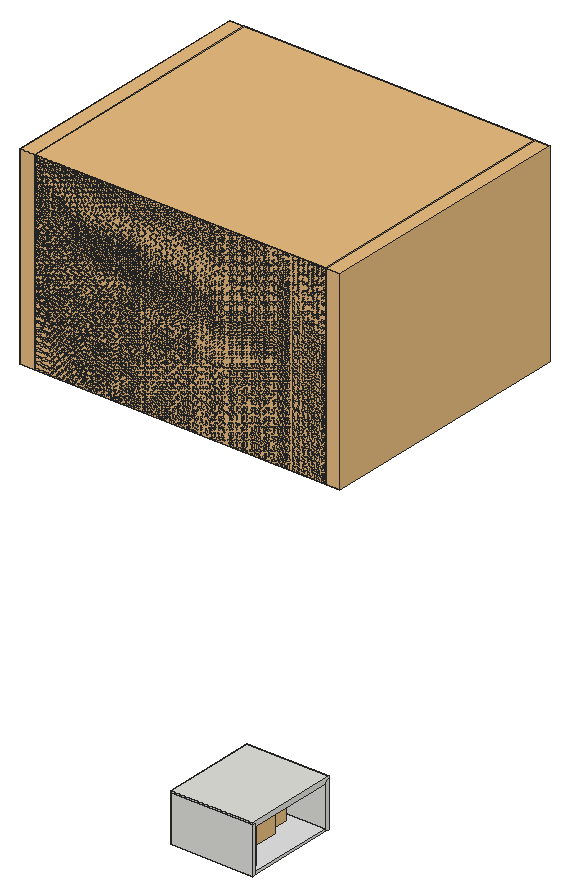
# SketchUp Ruby script. Lengths in inches.
U = 1.inch
M = Sketchup.active_model
def pt(a) = Geom::Point3d.new(a.map { |v| v * U })
def face(e, loops, mat)
  f = e.add_face(loops[0].map { |a| pt(a) })
  loops[1..].each { |l| e.add_face(l.map { |a| pt(a) }).erase! }
  f.material = f.back_material = mat if mat
  f
end
# faces: each face lists its corners as indices into pts; further lists are holes
def faces(e, pts, list, mat = nil) = list.each { |f| face(e, (f[0].is_a?(Array) ? f : [f]).map { |l| l.map { |i| pts[i] } }, mat) }
# xy, xz, yz: faces in a plane at the given z, y or x. An outline is a flat list of corners, or four numbers for a rectangle; further outlines are holes
def ring(l) = l.size == 4 ? [[l[0], l[1]], [l[2], l[1]], [l[2], l[3]], [l[0], l[3]]] : l.each_slice(2).to_a
def flat(e, list, mat, &to3) = list.each { |f| face(e, (f[0].is_a?(Array) ? f : [f]).map { |l| ring(l).map { |u, v| to3.(u, v) } }, mat) }
def xy(e, z, list, mat = nil) = flat(e, list, mat) { |x, y| [x, y, z] }
def xz(e, y, list, mat = nil) = flat(e, list, mat) { |x, z| [x, y, z] }
def yz(e, x, list, mat = nil) = flat(e, list, mat) { |y, z| [x, y, z] }
def lines(e, pts, list) = list.each { |a, b| e.add_line(pt(pts[a]), pt(pts[b])) }
# prism: a flat outline (further loops are holes) pulled along v
def prism(e, loops, v, mat = nil)
  f = face(e, loops, mat); d = Geom::Vector3d.new(v.map { |x| x * U })
  f.pushpull(f.normal.samedirection?(d) ? d.length : -d.length)
end
def box(e, o, s, mat = nil) = prism(e, [[o, [o[0] + s[0], o[1], o[2]], [o[0] + s[0], o[1] + s[1], o[2]], [o[0], o[1] + s[1], o[2]]]], [0, 0, s[2]], mat)
def at(x, y, z, deg = 0) = Geom::Transformation.translation(pt([x, y, z])) * Geom::Transformation.rotation(ORIGIN, Z_AXIS, deg.degrees)
def axes(o, x, y, z) = Geom::Transformation.new([*x, 0, *y, 0, *z, 0, *pt(o).to_a, 1])
def part(name) = M.definitions.add(name)
# library, detail: a bought-in or finely detailed component or shape, given as its bounding box
def library(name, o, s) = part(name).tap { |d| box(d.entities, o, s) }
def detail(e, o, s) = box(e.add_group.entities, o, s)
def put(e, d, t, mat = nil) = e.add_instance(d, t).tap { |i| i.material = mat if mat }
def group(e, t, mat = nil) = e.add_group.tap { |g| g.transformation = t; g.material = mat if mat }.entities
root = M.entities
M.materials.add("1466 AP 9476 Soft Whisper").color = [230, 233, 224]
M.materials.add("1472 AP 9469 Black Sea").color = [67, 75, 78]
M.materials.add("[Carrera Marble]").color = [207, 207, 207]
M.materials.add("[Granite Light Gray]").color = [49, 48, 47]
M.materials.add("[Marble Carrara Gold Floor Tile]").color = [229, 229, 229]
M.materials.add("[Stone Vein Gray]").color = [94, 94, 94]
M.materials.add("[Translucent Glass Blue]").color = [163, 215, 254]
M.materials.add("[Wood Veneer 01]").color = [83, 56, 38]
M.materials.add("[Wood Veneer 01]1").color = [74, 43, 22]
M.materials.add("[Wood Veneer 01]2").color = [120, 70, 37]
c1 = library("Object02",[-606.68,-655.71,-190.21],[1149.33,653.61,1636.06])
c2 = part("skp42")
put(c2.entities,c1,at(0,0,0))
c3 = part("Senza")
put(c3.entities,c2,at(-166.13,607.08,194.25))
c4 = library("kitchen+utensil",[-39.88,-27.4,0],[79.77,28.4,32.96])
c5 = library("1\#1",[-14.37,-13.42,0],[27.79,27.79,26.46])
c6 = library("ACCESS \#17",[0,0,0],[12.33,19.09,15.22])
c7 = library("AS-120-mm",[0,0,0],[63,4.72,48])
c8 = library("Potted Plant",[-13.58,-10.04,0],[38.83,39.25,67.18])
c9 = library("Mi & Gei Hardware - Brass Towel Ring",[0,0,0],[7.7,2.76,18.21])
c10 = library("DC3A\#1",[-17.72,-4.29,0],[35.44,8.58,13.65])
c11 = library("ILVE HP75C",[-22.61,-16.47,-1.74],[45.22,32.94,3.48])
c12 = library("11",[-1.9375,-1.9375,-28],[4,4,28])
c13 = library("Kitchen Tray Decor",[57.57,5.21,10.61],[18.31,18.31,13.72])
c14 = part("1")
box(c14.entities,[-20,0,0],[20,51,0.39])
c15 = library("2",[-1,-0.25,-0.25],[1,51.5,32.375])
c16 = part("5")
box(c16.entities,[0,-0.25,-0.25],[0.5,45,11.6875])
c17 = part("6")
box(c17.entities,[0,-0.25,-0.25],[0.5,45,15.9375])
c18 = library("תנור פולגור",[76.05,-2.36,7.75],[23.79,26.38,23.66])
c19 = library("\#1",[-189.34,-482.08,-290.58],[543.74,599.14,350.96])
c20 = part("Mixer\#1")
put(c20.entities,c19,at(-26.63,749.7,289.625))
c21 = library("ACCESS \#28",[0,0,-0.01],[22.01,8.97,21.09])
c22 = library("Kitchen+Sink",[0,0,-9.45],[39.37,19.69,22.29])
c23 = library("Drawer fronts",[0,0,0],[1.57,26.54,41.66])
c24 = library("French door refrigerator",[0,0,0],[35.5,29.25,69.5])
c25 = library("Group\#61",[-3.28,0,-3.2],[6.56,11.56,7.1])
c26 = library("Group1\#6",[-3.97,-4.36,4.58],[7.94,7.57,1.92])
c27 = library("Group2\#4",[-28.125,-19.52,30.85],[56.26,48.19,42.76])
c28 = part("215693")
put(c28.entities,c25,axes([0,0,0],[6.23163,0,0],[0,0,6.44624],[0,-6.23163,0]))
put(c28.entities,c26,axes([0,0.01,17.77],[2.3609,0,0],[0,2.52448,0],[0,0,1.96338]))
put(c28.entities,c27,axes([0.01,0.44,706.86],[14.88915,0,0],[0,14.88915,0],[0,0,12.38215]))
c29 = library("angular chimney",[0,0,0],[18.55,32.4,33.35])
c30 = library("oats",[14.82,-39.71,51.49],[19.78,4.73,8.06])
c31 = library("Group\#4",[0,0,0],[177,126,2])
c32 = library("Group\#6",[0,0,0],[0.5,124,34])
c33 = library("Group\#13",[0,0,0],[23.39,15.89,14.65])
c34 = library("Group\#43",[0,0,0],[27,126,29])
c35 = library("Group\#45",[0,0,-0.25],[18.5,126,21.25])
c36 = library("Group\#46",[0,0,-58.43],[152.74,148.09,107])
c37 = library("Group\#51",[0,0,0],[21.5,54,111])
c38 = library("Group\#53",[0,-18,0],[48,18,50])
c39 = library("Group\#59",[-5,-18,0],[6,18,71])
c40 = library("Group\#79",[0,-1,0],[23.9375,1,23.9375])
c41 = library("Group\#78",[0,0,-2.62],[198,180,7.62])
c42 = part("Group282\#1")
box(c42.entities,[-102,-4.5,0],[1,9,0.5])
c43 = part("Group283\#1")
box(c43.entities,[-100.5,-4.5,0],[1,9,0.5])
c44 = part("Group284\#1")
box(c44.entities,[-99,-4.5,0],[1,9,0.5])
c45 = part("Group285\#1")
box(c45.entities,[-97.5,-4.5,0],[1,9,0.5])
c46 = part("Group286\#1")
box(c46.entities,[-96,-4.5,0],[1,9,0.5])
c47 = part("Group287\#1")
box(c47.entities,[-94.5,-4.5,0],[1,9,0.5])
c48 = part("Group288\#1")
box(c48.entities,[-93,-4.5,0],[1,9,0.5])
c49 = part("Group289\#1")
box(c49.entities,[-91.5,-4.5,0],[1,9,0.5])
c50 = part("Group290\#1")
box(c50.entities,[-90,-4.5,0],[1,9,0.5])
c51 = part("Group291\#1")
box(c51.entities,[-88.5,-4.5,0],[1,9,0.5])
c52 = part("Group292\#1")
box(c52.entities,[-87,-4.5,0],[1,9,0.5])
c53 = part("Group293\#1")
box(c53.entities,[-85.5,-4.5,0],[1,9,0.5])
c54 = part("Group294\#1")
box(c54.entities,[-84,-4.5,0],[1,9,0.5])
c55 = part("Group295\#1")
box(c55.entities,[-82.5,-4.5,0],[1,9,0.5])
c56 = part("Group296\#1")
box(c56.entities,[-81,-4.5,0],[1,9,0.5])
c57 = part("Group297\#1")
box(c57.entities,[-79.5,-4.5,0],[1,9,0.5])
c58 = part("Group298\#1")
box(c58.entities,[-78,-4.5,0],[1,9,0.5])
c59 = part("Group299\#1")
box(c59.entities,[-76.5,-4.5,0],[1,9,0.5])
c60 = part("Group300\#1")
box(c60.entities,[-75,-4.5,0],[1,9,0.5])
c61 = part("Group301\#1")
box(c61.entities,[-73.5,-4.5,0],[1,9,0.5])
c62 = part("Group302\#1")
box(c62.entities,[-72,-4.5,0],[1,9,0.5])
c63 = part("Group303\#1")
box(c63.entities,[-70.5,-4.5,0],[1,9,0.5])
c64 = part("Group304\#1")
box(c64.entities,[-69,-4.5,0],[1,9,0.5])
c65 = part("Group305\#1")
box(c65.entities,[-67.5,-4.5,0],[1,9,0.5])
c66 = part("Group306\#1")
box(c66.entities,[-66,-4.5,0],[1,9,0.5])
c67 = part("Group307\#1")
box(c67.entities,[-64.5,-4.5,0],[1,9,0.5])
c68 = part("Group308\#1")
box(c68.entities,[-63,-4.5,0],[1,9,0.5])
c69 = part("Group309\#1")
box(c69.entities,[-61.5,-4.5,0],[1,9,0.5])
c70 = part("Group310\#1")
box(c70.entities,[-60,-4.5,0],[1,9,0.5])
c71 = part("Group311\#1")
box(c71.entities,[-58.5,-4.5,0],[1,9,0.5])
c72 = part("Group312\#1")
box(c72.entities,[-57,-4.5,0],[1,9,0.5])
c73 = part("Group313\#1")
box(c73.entities,[-55.5,-4.5,0],[1,9,0.5])
c74 = part("Group314\#1")
box(c74.entities,[-54,-4.5,0],[1,9,0.5])
c75 = part("Group315\#1")
box(c75.entities,[-52.5,-4.5,0],[1,9,0.5])
c76 = part("Group316\#1")
box(c76.entities,[-51,-4.5,0],[1,9,0.5])
c77 = part("Group317\#1")
box(c77.entities,[-49.5,-4.5,0],[1,9,0.5])
c78 = part("Group318\#1")
box(c78.entities,[-48,-4.5,0],[1,9,0.5])
c79 = part("Group319\#1")
box(c79.entities,[-46.5,-4.5,0],[1,9,0.5])
c80 = part("Group320\#1")
box(c80.entities,[-45,-4.5,0],[1,9,0.5])
c81 = part("Group321\#1")
box(c81.entities,[-43.5,-4.5,0],[1,9,0.5])
c82 = part("Group322\#1")
box(c82.entities,[-42,-4.5,0],[1,9,0.5])
c83 = part("Group323\#1")
box(c83.entities,[-40.5,-4.5,0],[1,9,0.5])
c84 = part("Group324\#1")
box(c84.entities,[-39,-4.5,0],[1,9,0.5])
c85 = part("Group325\#1")
box(c85.entities,[-37.5,-4.5,0],[1,9,0.5])
c86 = part("Group326\#1")
box(c86.entities,[-36,-4.5,0],[1,9,0.5])
c87 = part("Group327\#1")
box(c87.entities,[-34.5,-4.5,0],[1,9,0.5])
c88 = part("Group328\#1")
box(c88.entities,[-33,-4.5,0],[1,9,0.5])
c89 = part("Group329\#1")
box(c89.entities,[-31.5,-4.5,0],[1,9,0.5])
c90 = part("Group330\#1")
box(c90.entities,[-30,-4.5,0],[1,9,0.5])
c91 = part("Group331\#1")
box(c91.entities,[-28.5,-4.5,0],[1,9,0.5])
c92 = part("Group332\#1")
box(c92.entities,[-27,-4.5,0],[1,9,0.5])
c93 = part("Group333\#1")
box(c93.entities,[-25.5,-4.5,0],[1,9,0.5])
c94 = part("Group334\#1")
box(c94.entities,[-24,-4.5,0],[1,9,0.5])
c95 = part("Group335\#1")
box(c95.entities,[-22.5,-4.5,0],[1,9,0.5])
c96 = part("Group336\#1")
box(c96.entities,[-21,-4.5,0],[1,9,0.5])
c97 = part("Group337\#1")
box(c97.entities,[-19.5,-4.5,0],[1,9,0.5])
c98 = part("Group338\#1")
box(c98.entities,[-18,-4.5,0],[1,9,0.5])
c99 = part("Group339\#1")
box(c99.entities,[-16.5,-4.5,0],[1,9,0.5])
c100 = part("Group340\#1")
box(c100.entities,[-15,-4.5,0],[1,9,0.5])
c101 = part("Group341\#1")
box(c101.entities,[-13.5,-4.5,0],[1,9,0.5])
c102 = part("Group342\#1")
box(c102.entities,[-12,-4.5,0],[1,9,0.5])
c103 = part("Group343\#1")
box(c103.entities,[-10.5,-4.5,0],[1,9,0.5])
c104 = part("Group344\#1")
box(c104.entities,[-9,-4.5,0],[1,9,0.5])
c105 = part("Group345\#1")
box(c105.entities,[-7.5,-4.5,0],[1,9,0.5])
c106 = part("Group346\#1")
box(c106.entities,[-6,-4.5,0],[1,9,0.5])
c107 = part("Group347\#1")
box(c107.entities,[-4.5,-4.5,0],[1,9,0.5])
c108 = part("Group348\#1")
box(c108.entities,[-3,-4.5,0],[1,9,0.5])
c109 = part("Group349\#1")
box(c109.entities,[-1.5,-4.5,0],[1,9,0.5])
c110 = part("Group350\#1")
box(c110.entities,[0,-4.5,0],[1,9,0.5])
c111 = part("Group351\#1")
box(c111.entities,[1.5,-4.5,0],[1,9,0.5])
c112 = part("Group352\#1")
box(c112.entities,[3,-4.5,0],[1,9,0.5])
c113 = part("Group353\#1")
box(c113.entities,[4.5,-4.5,0],[1,9,0.5])
c114 = part("Group354\#1")
box(c114.entities,[6,-4.5,0],[1,9,0.5])
c115 = part("Group355\#1")
box(c115.entities,[7.5,-4.5,0],[1,9,0.5])
c116 = part("Group356\#1")
box(c116.entities,[9,-4.5,0],[1,9,0.5])
c117 = part("Group357\#1")
box(c117.entities,[10.5,-4.5,0],[1,9,0.5])
c118 = part("Group358\#1")
box(c118.entities,[12,-4.5,0],[1,9,0.5])
c119 = part("Group359\#1")
box(c119.entities,[13.5,-4.5,0],[1,9,0.5])
c120 = part("Group360\#1")
box(c120.entities,[15,-4.5,0],[1,9,0.5])
c121 = part("Group361\#1")
box(c121.entities,[16.5,-4.5,0],[1,9,0.5])
c122 = part("Group362\#1")
box(c122.entities,[18,-4.5,0],[1,9,0.5])
c123 = part("Group363\#1")
box(c123.entities,[19.5,-4.5,0],[1,9,0.5])
c124 = part("Group364\#1")
box(c124.entities,[21,-4.5,0],[1,9,0.5])
c125 = part("Group365\#1")
box(c125.entities,[22.5,-4.5,0],[1,9,0.5])
c126 = part("Group366\#1")
box(c126.entities,[24,-4.5,0],[1,9,0.5])
c127 = part("Group367\#1")
box(c127.entities,[25.5,-4.5,0],[1,9,0.5])
c128 = part("Group368\#1")
box(c128.entities,[27,-4.5,0],[1,9,0.5])
c129 = part("Group369\#1")
box(c129.entities,[28.5,-4.5,0],[1,9,0.5])
c130 = part("Group370\#1")
box(c130.entities,[30,-4.5,0],[1,9,0.5])
c131 = part("Group371\#1")
box(c131.entities,[31.5,-4.5,0],[1,9,0.5])
c132 = part("Group372\#1")
box(c132.entities,[33,-4.5,0],[1,9,0.5])
c133 = part("Group373\#1")
box(c133.entities,[34.5,-4.5,0],[1,9,0.5])
c134 = part("Group374\#1")
box(c134.entities,[36,-4.5,0],[1,9,0.5])
c135 = part("Group375\#1")
box(c135.entities,[37.5,-4.5,0],[1,9,0.5])
c136 = part("Group376\#1")
box(c136.entities,[39,-4.5,0],[1,9,0.5])
c137 = part("Group377\#1")
box(c137.entities,[40.5,-4.5,0],[1,9,0.5])
c138 = part("Group378\#1")
box(c138.entities,[42,-4.5,0],[1,9,0.5])
c139 = part("Group379\#1")
box(c139.entities,[43.5,-4.5,0],[1,9,0.5])
c140 = part("Group380\#1")
box(c140.entities,[45,-4.5,0],[1,9,0.5])
c141 = part("Group381\#1")
box(c141.entities,[46.5,-4.5,0],[1,9,0.5])
c142 = part("Group382\#1")
box(c142.entities,[48,-4.5,0],[1,9,0.5])
c143 = part("Group383\#1")
box(c143.entities,[49.5,-4.5,0],[1,9,0.5])
c144 = part("Group384\#1")
box(c144.entities,[51,-4.5,0],[1,9,0.5])
c145 = part("Group385\#1")
box(c145.entities,[52.5,-4.5,0],[1,9,0.5])
c146 = part("Group386\#1")
box(c146.entities,[54,-4.5,0],[1,9,0.5])
c147 = part("Group387\#1")
box(c147.entities,[55.5,-4.5,0],[1,9,0.5])
c148 = part("Group388\#1")
box(c148.entities,[57,-4.5,0],[1,9,0.5])
c149 = part("Group389\#1")
box(c149.entities,[58.5,-4.5,0],[1,9,0.5])
c150 = part("Group390\#1")
box(c150.entities,[60,-4.5,0],[1,9,0.5])
c151 = part("Group391\#1")
box(c151.entities,[61.5,-4.5,0],[1,9,0.5])
c152 = part("Group392\#1")
box(c152.entities,[63,-4.5,0],[1,9,0.5])
c153 = part("Group393\#1")
box(c153.entities,[64.5,-4.5,0],[1,9,0.5])
c154 = part("Group394\#1")
box(c154.entities,[66,-4.5,0],[1,9,0.5])
c155 = part("Group395\#1")
box(c155.entities,[67.5,-4.5,0],[1,9,0.5])
c156 = part("Group396\#1")
box(c156.entities,[69,-4.5,0],[1,9,0.5])
c157 = part("Group397\#1")
box(c157.entities,[70.5,-4.5,0],[1,9,0.5])
c158 = part("Group398\#1")
box(c158.entities,[72,-4.5,0],[1,9,0.5])
c159 = part("Group399\#1")
box(c159.entities,[73.5,-4.5,0],[1,9,0.5])
c160 = part("Group400\#1")
box(c160.entities,[75,-4.5,0],[1,9,0.5])
c161 = part("Group401\#1")
box(c161.entities,[76.5,-4.5,0],[1,9,0.5])
c162 = part("Group402\#1")
box(c162.entities,[78,-4.5,0],[1,9,0.5])
c163 = part("Group403\#1")
box(c163.entities,[79.5,-4.5,0],[1,9,0.5])
c164 = part("Group404\#1")
box(c164.entities,[81,-4.5,0],[1,9,0.5])
c165 = part("Group405\#1")
box(c165.entities,[82.5,-4.5,0],[1,9,0.5])
c166 = part("Group406\#1")
box(c166.entities,[84,-4.5,0],[1,9,0.5])
c167 = part("Group407\#1")
box(c167.entities,[85.5,-4.5,0],[1,9,0.5])
c168 = part("Group408\#1")
box(c168.entities,[87,-4.5,0],[1,9,0.5])
c169 = part("Group409\#1")
box(c169.entities,[88.5,-4.5,0],[1,9,0.5])
c170 = part("Group410\#1")
box(c170.entities,[90,-4.5,0],[1,9,0.5])
c171 = part("Group411\#1")
box(c171.entities,[91.5,-4.5,0],[1,9,0.5])
c172 = part("Group412\#1")
box(c172.entities,[93,-4.5,0],[1,9,0.5])
c173 = part("Group413\#1")
box(c173.entities,[94.5,-4.5,0],[1,9,0.5])
c174 = part("Group414\#1")
box(c174.entities,[96,-4.5,0],[1,9,0.5])
c175 = part("Group415\#1")
box(c175.entities,[97.5,-4.5,0],[1,9,0.5])
c176 = part("Group416\#1")
box(c176.entities,[99,-4.5,0],[1,9,0.5])
c177 = part("Group417\#1")
box(c177.entities,[100.5,-4.5,0],[1,9,0.5])
c178 = part("Group280\#1")
put(c178.entities,c42,at(0,0,0))
put(c178.entities,c43,at(0,0,0))
put(c178.entities,c44,at(0,0,0))
put(c178.entities,c45,at(0,0,0))
put(c178.entities,c46,at(0,0,0))
put(c178.entities,c47,at(0,0,0))
put(c178.entities,c48,at(0,0,0))
put(c178.entities,c49,at(0,0,0))
put(c178.entities,c50,at(0,0,0))
put(c178.entities,c51,at(0,0,0))
put(c178.entities,c52,at(0,0,0))
put(c178.entities,c53,at(0,0,0))
put(c178.entities,c54,at(0,0,0))
put(c178.entities,c55,at(0,0,0))
put(c178.entities,c56,at(0,0,0))
put(c178.entities,c57,at(0,0,0))
put(c178.entities,c58,at(0,0,0))
put(c178.entities,c59,at(0,0,0))
put(c178.entities,c60,at(0,0,0))
put(c178.entities,c61,at(0,0,0))
put(c178.entities,c62,at(0,0,0))
put(c178.entities,c63,at(0,0,0))
put(c178.entities,c64,at(0,0,0))
put(c178.entities,c65,at(0,0,0))
put(c178.entities,c66,at(0,0,0))
put(c178.entities,c67,at(0,0,0))
put(c178.entities,c68,at(0,0,0))
put(c178.entities,c69,at(0,0,0))
put(c178.entities,c70,at(0,0,0))
put(c178.entities,c71,at(0,0,0))
put(c178.entities,c72,at(0,0,0))
put(c178.entities,c73,at(0,0,0))
put(c178.entities,c74,at(0,0,0))
put(c178.entities,c75,at(0,0,0))
put(c178.entities,c76,at(0,0,0))
put(c178.entities,c77,at(0,0,0))
put(c178.entities,c78,at(0,0,0))
put(c178.entities,c79,at(0,0,0))
put(c178.entities,c80,at(0,0,0))
put(c178.entities,c81,at(0,0,0))
put(c178.entities,c82,at(0,0,0))
put(c178.entities,c83,at(0,0,0))
put(c178.entities,c84,at(0,0,0))
put(c178.entities,c85,at(0,0,0))
put(c178.entities,c86,at(0,0,0))
put(c178.entities,c87,at(0,0,0))
put(c178.entities,c88,at(0,0,0))
put(c178.entities,c89,at(0,0,0))
put(c178.entities,c90,at(0,0,0))
put(c178.entities,c91,at(0,0,0))
put(c178.entities,c92,at(0,0,0))
put(c178.entities,c93,at(0,0,0))
put(c178.entities,c94,at(0,0,0))
put(c178.entities,c95,at(0,0,0))
put(c178.entities,c96,at(0,0,0))
put(c178.entities,c97,at(0,0,0))
put(c178.entities,c98,at(0,0,0))
put(c178.entities,c99,at(0,0,0))
put(c178.entities,c100,at(0,0,0))
put(c178.entities,c101,at(0,0,0))
put(c178.entities,c102,at(0,0,0))
put(c178.entities,c103,at(0,0,0))
put(c178.entities,c104,at(0,0,0))
put(c178.entities,c105,at(0,0,0))
put(c178.entities,c106,at(0,0,0))
put(c178.entities,c107,at(0,0,0))
put(c178.entities,c108,at(0,0,0))
put(c178.entities,c109,at(0,0,0))
put(c178.entities,c110,at(0,0,0))
put(c178.entities,c111,at(0,0,0))
put(c178.entities,c112,at(0,0,0))
put(c178.entities,c113,at(0,0,0))
put(c178.entities,c114,at(0,0,0))
put(c178.entities,c115,at(0,0,0))
put(c178.entities,c116,at(0,0,0))
put(c178.entities,c117,at(0,0,0))
put(c178.entities,c118,at(0,0,0))
put(c178.entities,c119,at(0,0,0))
put(c178.entities,c120,at(0,0,0))
put(c178.entities,c121,at(0,0,0))
put(c178.entities,c122,at(0,0,0))
put(c178.entities,c123,at(0,0,0))
put(c178.entities,c124,at(0,0,0))
put(c178.entities,c125,at(0,0,0))
put(c178.entities,c126,at(0,0,0))
put(c178.entities,c127,at(0,0,0))
put(c178.entities,c128,at(0,0,0))
put(c178.entities,c129,at(0,0,0))
put(c178.entities,c130,at(0,0,0))
put(c178.entities,c131,at(0,0,0))
put(c178.entities,c132,at(0,0,0))
put(c178.entities,c133,at(0,0,0))
put(c178.entities,c134,at(0,0,0))
put(c178.entities,c135,at(0,0,0))
put(c178.entities,c136,at(0,0,0))
put(c178.entities,c137,at(0,0,0))
put(c178.entities,c138,at(0,0,0))
put(c178.entities,c139,at(0,0,0))
put(c178.entities,c140,at(0,0,0))
put(c178.entities,c141,at(0,0,0))
put(c178.entities,c142,at(0,0,0))
put(c178.entities,c143,at(0,0,0))
put(c178.entities,c144,at(0,0,0))
put(c178.entities,c145,at(0,0,0))
put(c178.entities,c146,at(0,0,0))
put(c178.entities,c147,at(0,0,0))
put(c178.entities,c148,at(0,0,0))
put(c178.entities,c149,at(0,0,0))
put(c178.entities,c150,at(0,0,0))
put(c178.entities,c151,at(0,0,0))
put(c178.entities,c152,at(0,0,0))
put(c178.entities,c153,at(0,0,0))
put(c178.entities,c154,at(0,0,0))
put(c178.entities,c155,at(0,0,0))
put(c178.entities,c156,at(0,0,0))
put(c178.entities,c157,at(0,0,0))
put(c178.entities,c158,at(0,0,0))
put(c178.entities,c159,at(0,0,0))
put(c178.entities,c160,at(0,0,0))
put(c178.entities,c161,at(0,0,0))
put(c178.entities,c162,at(0,0,0))
put(c178.entities,c163,at(0,0,0))
put(c178.entities,c164,at(0,0,0))
put(c178.entities,c165,at(0,0,0))
put(c178.entities,c166,at(0,0,0))
put(c178.entities,c167,at(0,0,0))
put(c178.entities,c168,at(0,0,0))
put(c178.entities,c169,at(0,0,0))
put(c178.entities,c170,at(0,0,0))
put(c178.entities,c171,at(0,0,0))
put(c178.entities,c172,at(0,0,0))
put(c178.entities,c173,at(0,0,0))
put(c178.entities,c174,at(0,0,0))
put(c178.entities,c175,at(0,0,0))
put(c178.entities,c176,at(0,0,0))
put(c178.entities,c177,at(0,0,0))
g1 = group(root,at(225,9,0,90))
put(g1,c3,axes([202.64,193.52,-0.13],[0.03318,0,0],[0,0.03716,0],[0,0,0.03318]))
put(g1,c4,axes([0.42,103.56,40],[0,0.34,0],[-0.34,0,0],[0,0,0.34]))
put(g1,c5,axes([133.34,206.44,40],[0.66,0,0],[0,0.66,0],[0,0,0.66]))
put(g1,c6,axes([0.08,195.96,40],[1,0,0],[0,-1,0],[0,0,1]))
g2 = group(g1,at(-9,0,0))
xy(g2,-6,[[0,0,0,225,261,225,261,0,252,0,252,216,9,216,9,0]])
xy(g2,0,[[9,69,9,216,186,216,186,91,168,91,168,200,25,200,25,69]])
xy(g2,4,[[9,69,25,69,25,200,168,200,168,91,186,91,186,216,9,216]])
xy(g2,49,[[39,216,102,225]])
xy(g2,97,[[39,216,102,225]])
xy(g2,120,[[0,0,9,0,9,216,252,216,252,0,261,0,261,225,0,225]])
xz(g2,0,[[0,-6,9,120],[252,-6,261,120]])
xz(g2,69,[[9,0,25,4]])
xz(g2,91,[[168,0,186,4]],"[Granite Light Gray]")
xz(g2,200,[[25,0,168,4]],"[Granite Light Gray]")
xz(g2,216,[[[9,-6,252,-6,252,120,9,120,9,4,186,4,186,0,9,0],[39,49,102,97]]],"1466 AP 9476 Soft Whisper")
xz(g2,225,[[[0,-6,261,120],[39,49,102,97]]])
yz(g2,0,[[0,-6,225,120]])
yz(g2,9,[[0,-6,216,0]])
yz(g2,9,[[0,0,69,0,69,4,216,4,216,120,0,120]],"1466 AP 9476 Soft Whisper")
yz(g2,25,[[69,0,200,4]],"[Granite Light Gray]")
yz(g2,39,[[216,49,225,97]])
yz(g2,102,[[216,49,225,97]])
yz(g2,168,[[91,0,200,4]],"[Granite Light Gray]")
yz(g2,186,[[91,0,216,4]],"[Granite Light Gray]")
yz(g2,252,[[0,-6,216,120]])
yz(g2,261,[[0,-6,225,120]])
put(g2,c7,axes([39,223.6,49],[1,0,0],[0,-1,0],[0,0,1]))
put(g2,c8,axes([234.52,192.4375,0],[0.83,0,0],[0,0.83,0],[0,0,0.83]))
put(g2,c9,at(221.93,209.6,47.19))
put(g2,c10,axes([22.48,122.06,62],[0,-0.5612,0],[0.5612,0,0],[0,0,0.5612]))
put(g2,c11,axes([20.61,151.42,41.22],[0,-0.7,0],[-0.7,0,0],[0,0,0.7]))
put(g2,c12,at(178.01,98.35,112.83))
put(g2,c12,at(178.01,116.35,112.83))
put(g2,c12,at(178.01,134.35,112.83))
put(g2,c13,at(95.99,192.4,29.39))
g3 = group(g2,at(9,90,4),"[Carrera Marble]")
xy(g3,0,[[0,0,0,126,177,126,177,125,175.5,125,175.5,1,177,1,177,0,153,0,153,105,21,105,21,0]])
xy(g3,1.0625,[[1,1,21,45.5],[153,1,174,52],[1,46.5,21,91],[153,53,174,53,174,125,154,125,154,104,153,104],[1,92,21,104],
  [22,105,43,105,43,125,1,125,1,106,22,106],[44,105,79.5,125],[116.5,105,152,125]])
xy(g3,1.0625,[[80.5,105,115.5,125]],"[Wood Veneer 01]1")
xy(g3,10.0625,[[44,106,79.5,125]])
xy(g3,11.0625,[[44,106,79.5,125]])
xy(g3,12.25,[[1,1,21,45.5]])
xy(g3,13.25,[[1,1,21,45.5]])
xy(g3,16.5,[[1,46.5,21,91],[80.5,105,115.5,125],[1,106,43,125]])
xy(g3,17.5,[[1,46.5,21,91],[1,106,43,125]])
xy(g3,17.5,[[80.5,105,115.5,125]],"[Wood Veneer 01]1")
xy(g3,24.4375,[[1,1,21,45.5]])
xy(g3,25.4375,[[1,1,21,45.5]])
xy(g3,32.9375,[[1,1,21,45.5],[153,1,174,52],[1,46.5,21,91],[153,53,153,104,154,104,154,125,174,125,174,53],[1,92,21,104],
  [22,105,22,106,1,106,1,125,43,125,43,105],[[44,105,79.5,125],[47,107,76.5,123]],[80.5,105,115.5,125],[116.5,105,152,125]])
xy(g3,34,[[[0,0,21,0,21,105,153,105,153,0,177,0,177,1,175.5,1,175.5,125,177,125,177,126,0,126],[47,107,76.5,123]]])
xz(g3,0,[[0,0,21,34],[153,0,177,34]])
xz(g3,1,[[175.5,0,177,34],[1,1.0625,21,12.25],[153,1.0625,174,32.9375],[1,13.25,21,24.4375],[1,25.4375,21,32.9375]])
xz(g3,45.5,[[1,1.0625,21,12.25],[1,13.25,21,24.4375],[1,25.4375,21,32.9375]])
xz(g3,46.5,[[1,1.0625,21,16.5],[1,17.5,21,32.9375]])
xz(g3,52,[[153,1.0625,174,32.9375]])
xz(g3,53,[[153,1.0625,174,32.9375]])
xz(g3,91,[[1,1.0625,21,16.5],[1,17.5,21,32.9375]])
xz(g3,92,[[1,1.0625,21,32.9375]])
xz(g3,104,[[1,1.0625,21,32.9375],[153,1.0625,154,32.9375]])
xz(g3,105,[[[21,0,153,34],[44,1.0625,79.5,32.9375],[116.5,1.0625,152,32.9375],[22,1.0625,43,32.9375],[80.5,17.5,115.5,32.9375],[80.5,1.0625,115.5,16.5]]],"[Wood Veneer 01]1")
xz(g3,106,[[1,1.0625,22,16.5],[44,10.0625,79.5,11.0625],[1,16.5,22,17.5],[22,16.5,43,17.5],[1,17.5,22,32.9375]])
xz(g3,107,[[47,32.9375,76.5,34]])
xz(g3,123,[[47,32.9375,76.5,34]])
xz(g3,125,[[175.5,0,177,34],[1,1.0625,43,16.5],[44,1.0625,79.5,10.0625],[116.5,1.0625,152,32.9375],[154,1.0625,174,32.9375],
  [44,11.0625,79.5,32.9375],[1,17.5,43,32.9375]])
xz(g3,125,[[80.5,1.0625,115.5,16.5],[80.5,17.5,115.5,32.9375]],"[Wood Veneer 01]1")
xz(g3,126,[[0,0,177,34]])
yz(g3,0,[[0,0,126,34]])
yz(g3,1,[[1,1.0625,45.5,12.25],[46.5,1.0625,91,16.5],[92,1.0625,104,32.9375],[106,1.0625,125,16.5],[1,13.25,45.5,24.4375],
  [46.5,17.5,91,32.9375],[106,17.5,125,32.9375],[1,25.4375,45.5,32.9375]])
yz(g3,21,[[[0,0,105,34],[46.5,17.5,91,32.9375],[46.5,1.0625,91,16.5],[1,13.25,45.5,24.4375],[1,1.0625,45.5,12.25],[92,1.0625,104,32.9375],[1,25.4375,45.5,32.9375]]],"[Wood Veneer 01]1")
yz(g3,22,[[105,1.0625,106,32.9375]])
yz(g3,43,[[105,1.0625,105,32.9375,125,32.9375,125,17.5,106,17.5,106,16.5,125,16.5,125,1.0625]])
yz(g3,44,[[105,1.0625,125,1.0625,125,10.0625,106,10.0625,106,11.0625,125,11.0625,125,32.9375,105,32.9375]])
yz(g3,47,[[107,32.9375,123,34]])
yz(g3,76.5,[[107,32.9375,123,34]])
yz(g3,79.5,[[105,1.0625,105,32.9375,125,32.9375,125,11.0625,106,11.0625,106,10.0625,125,10.0625,125,1.0625]])
yz(g3,80.5,[[105,1.0625,125,16.5],[105,17.5,125,32.9375]],"[Wood Veneer 01]1")
yz(g3,115.5,[[105,1.0625,125,16.5],[105,17.5,125,32.9375]],"[Wood Veneer 01]1")
yz(g3,116.5,[[105,1.0625,125,32.9375]])
yz(g3,152,[[105,1.0625,125,32.9375]])
yz(g3,153,[[[0,0,105,34],[53,1.0625,104,32.9375],[1,1.0625,52,32.9375]]])
yz(g3,154,[[104,1.0625,125,32.9375]])
yz(g3,174,[[1,1.0625,52,32.9375],[53,1.0625,125,32.9375]])
yz(g3,175.5,[[1,0,125,34]])
yz(g3,177,[[0,0,1,34],[125,0,126,34]])
put(g3,c14,axes([174,1,11.55],[1,0,0],[0,1,0],[0,0,1.0625]),"[Translucent Glass Blue]")
put(g3,c14,axes([174,1,22.03],[1,0,0],[0,1,0],[0,0,1.0625]),"[Translucent Glass Blue]")
put(g3,c14,axes([174,53,22.03],[1,0,0],[0,1.41176,0],[0,0,1.0625]),"[Translucent Glass Blue]")
put(g3,c14,axes([174,53,11.55],[1,0,0],[0,1.41176,0],[0,0,1.0625]),"[Translucent Glass Blue]")
put(g3,c15,at(153,53,1.0625),"[Wood Veneer 01]")
put(g3,c15,at(153,1,1.0625),"[Wood Veneer 01]")
put(g3,c16,at(21,1,13.25),"1472 AP 9469 Black Sea")
put(g3,c16,at(21,1,1.0625),"1472 AP 9469 Black Sea")
put(g3,c17,at(21,46.5,17.5),"1472 AP 9469 Black Sea")
put(g3,c17,at(21,46.5,1.0625),"1472 AP 9469 Black Sea")
put(g3,c18,axes([1.14,105.1,-9.38],[1.51685,0,0],[0,0.82878,0],[0,0,1.34715]))
put(g3,c20,axes([113.75,117.13,1.1],[0.0007,-0.03626,0],[-0.03775,-0.00072,0],[0,0,0.03842]))
put(g3,c21,axes([93.08,105,1.0625],[0.7992,0,0],[0,1,0],[0,0,0.73236]))
put(g3,c22,at(46.68,104.53,36))
put(g3,c23,axes([19.71,-20,19.79],[0.82,0,0],[0,0.71577,0],[0,0,0.8692]))
put(g3,c24,axes([1,-74,-4],[0,1.46479,0],[0.65065,0,0],[0,0,1.09353]))
put(g3,c28,at(197.17,21.25,-3.99,-90))
put(g3,c28,at(197.17,61.875,-3.99,-90))
put(g3,c29,axes([0.08,44.79,57],[0.99328,0,0],[0,1,0],[0,0,0.83947]))
put(g3,c30,at(49.48,35.82,6.51,-90))
put(g3,c31,at(0,0,34),"[Carrera Marble]")
put(g3,c32,at(175.5,1,0))
g4 = group(g3,at(21,1,25.4375),"1472 AP 9469 Black Sea")
box(g4,[0,-0.25,-0.25],[0.5,45,8])
g5 = group(g3,at(21,92,1.0625),"1472 AP 9469 Black Sea")
box(g5,[0,-0.25,-0.25],[0.5,12.5,32.375])
g6 = group(g3,at(22,105,1.0625),"1472 AP 9469 Black Sea")
box(g6,[-0.25,-0.5,-0.25],[21.5,0.5,32.375])
g7 = group(g3,at(44,105,1.0625),"1472 AP 9469 Black Sea")
box(g7,[-0.25,-0.5,-0.25],[17.95,0.5,32.375])
box(g7,[17.8,-0.5,-0.25],[17.95,0.5,32.375])
# 1 loose lines left out
put(g3,c33,axes([82.625,105,17.5],[1.33,0,0],[0,1,0],[0,0,1.05407]))
put(g3,c34,at(0,0,57),"[Wood Veneer 01]1")
put(g3,c35,at(0,0,86),"[Wood Veneer 01]1")
put(g3,c36,at(0,-21,58.43),"1472 AP 9469 Black Sea")
put(g3,c37,at(0,-75,-4))
put(g3,c38,at(109,126,57),"[Wood Veneer 01]")
put(g3,c39,at(176,126,36),"[Wood Veneer 01]")
g8 = group(g2,at(9,90,40))
xy(g8,0,[[0,0,0.08,125.92],[0,125.92,171,126]],"[Stone Vein Gray]")
xy(g8,9,[[30,125.92,93,126]],"[Stone Vein Gray]")
xy(g8,22,[[0,0,0.08,43],[0,79,0.08,125.92],[0,125.92,30,126],[93,125.92,171,126]],"[Stone Vein Gray]")
xy(g8,49,[[0,43,0.08,79]],"[Stone Vein Gray]")
xz(g8,0,[[0,0,0.08,22]],"[Stone Vein Gray]")
xz(g8,43,[[0,22,0.08,49]],"[Stone Vein Gray]")
xz(g8,79,[[0,22,0.08,49]],"[Stone Vein Gray]")
xz(g8,125.92,[[0.08,0,171,0,171,22,93,22,93,9,30,9,30,22,0.08,22]],"[Stone Vein Gray]")
xz(g8,126,[[0,0,0,22,30,22,30,9,93,9,93,22,171,22,171,0]],"[Stone Vein Gray]")
yz(g8,0.08,[[0,0,125.92,0,125.92,22,79,22,79,49,43,49,43,22,0,22]],"[Stone Vein Gray]")
yz(g8,30,[[125.92,9,126,22]],"[Stone Vein Gray]")
yz(g8,93,[[125.92,9,126,22]],"[Stone Vein Gray]")
yz(g8,171,[[125.92,0,126,22]],"[Stone Vein Gray]")
put(g2,c40,axes([193.03,215,49.95],[1,0,0],[0,1,0],[0,0,1.4]))
g9 = group(g1,at(0,0,-6))
xy(g9,0,[[0,0,243,216]])
xy(g9,6,[[0,0,243,216]],"[Marble Carrara Gold Floor Tile]")
xz(g9,0,[[0,0,243,6]])
xz(g9,216,[[0,0,243,6]])
yz(g9,0,[[0,0,216,6]])
yz(g9,243,[[0,0,216,6]])
g10 = group(g1,at(-9,0,120))
xy(g10,-9,[[[9,0,261,225],[30,12,252,216]]])
xy(g10,0,[[0,0,9,225],[[30,12,252,216],[66,180,66.0625,180,66,180]],[66,180,66.0625,180,66,180]])
xy(g10,6,[[0,0,261,225]])
xz(g10,0,[[9,-9,261,-9,261,6,0,6,0,0,9,0]])
xz(g10,12,[[30,-9,252,0]])
xz(g10,216,[[30,-9,252,0]])
xz(g10,225,[[9,-9,9,0,0,0,0,6,261,6,261,-9]])
yz(g10,0,[[0,0,225,6]])
yz(g10,9,[[0,-9,225,0]])
yz(g10,30,[[12,-9,216,0]])
yz(g10,252,[[12,-9,216,0]])
yz(g10,261,[[0,-9,225,6]])
# 7 loose lines left out
put(g10,c41,axes([42,24,-9],[1,0,0],[0,1,0],[0,0,1.8]))
put(g10,c178,axes([30,114,-4.5],[0,1,0],[0,0,1],[1,0,0]),"[Wood Veneer 01]2")
